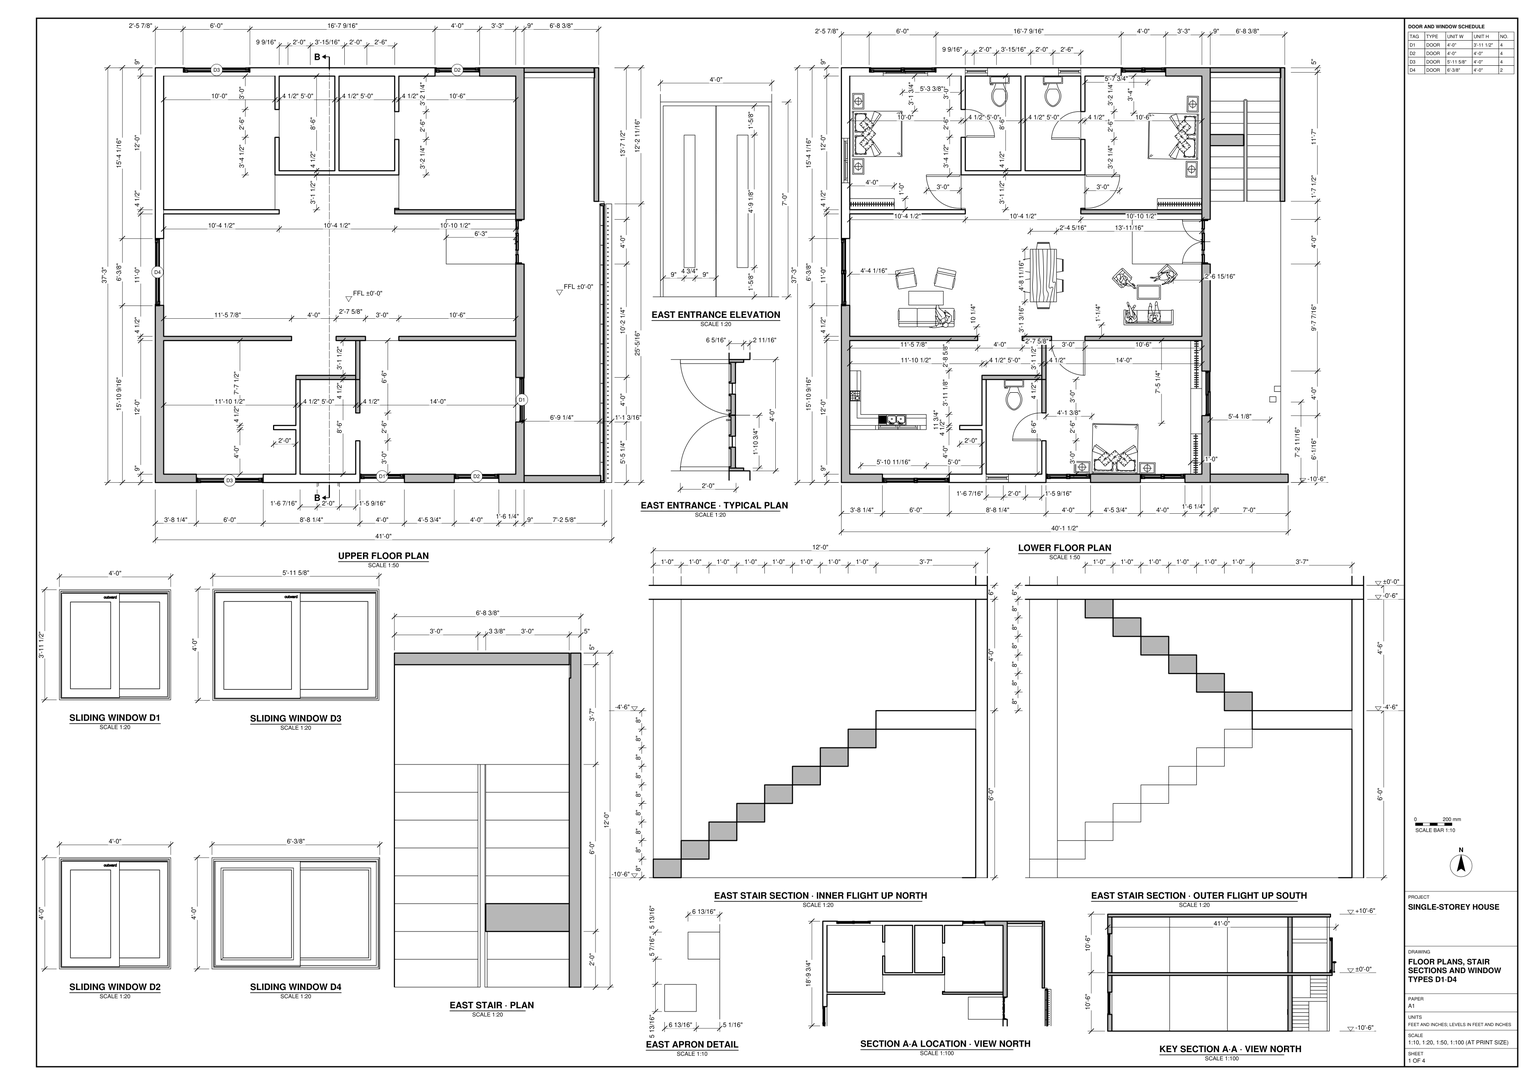
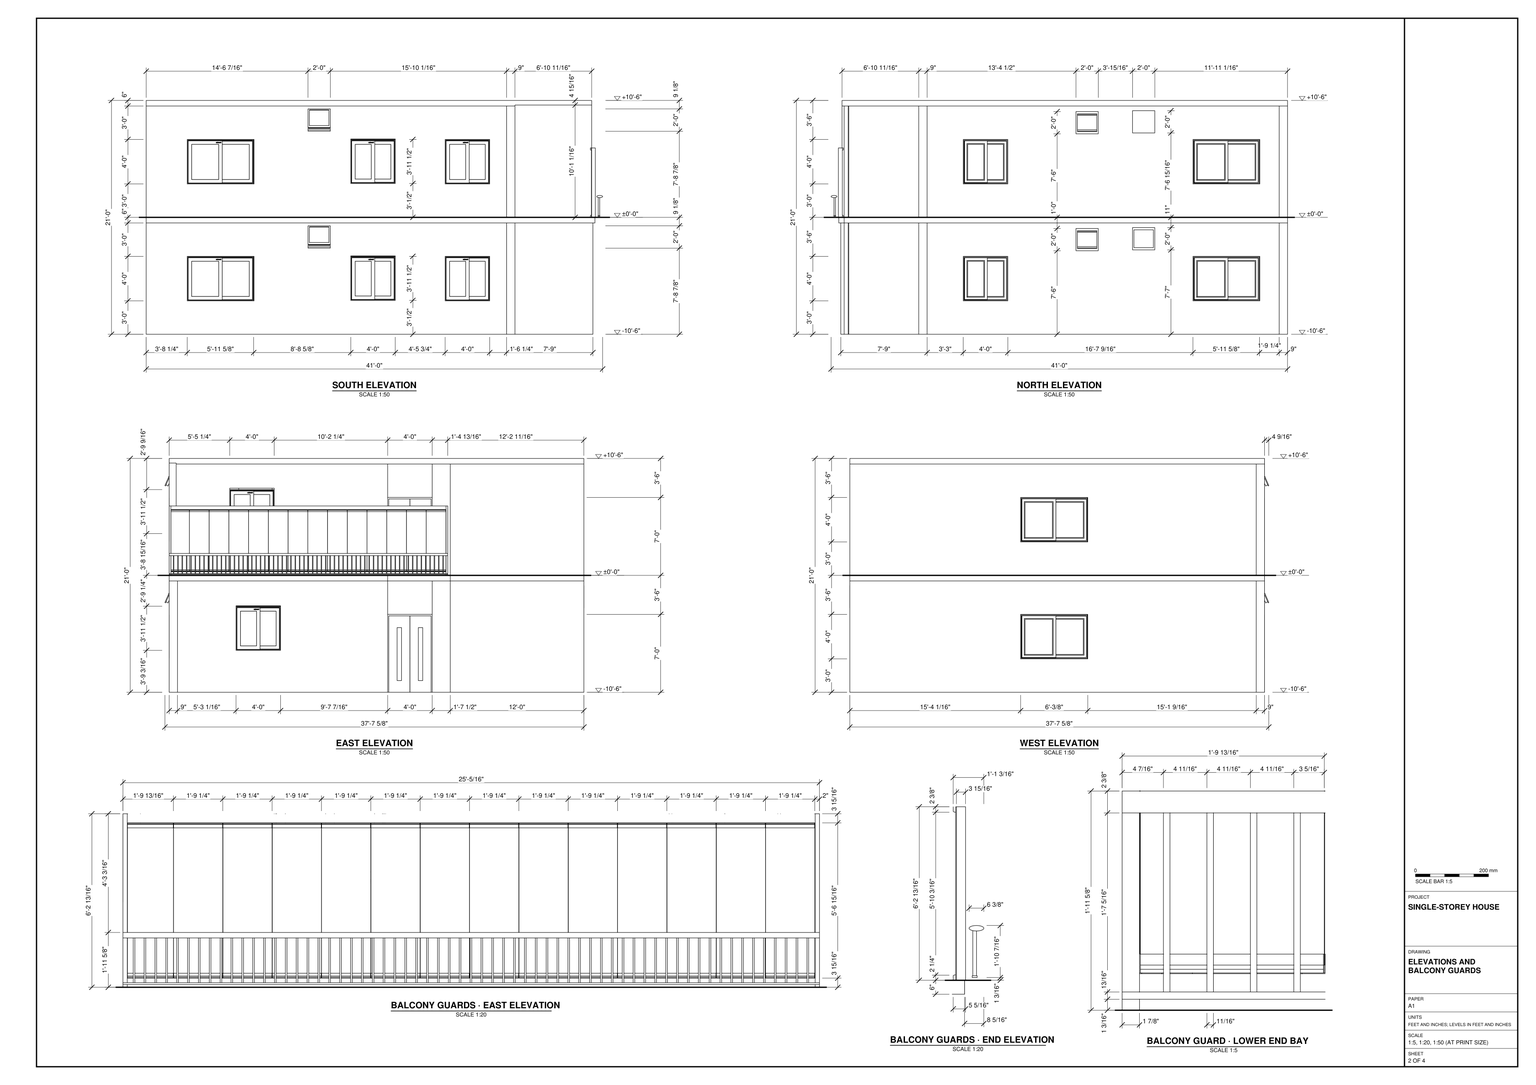
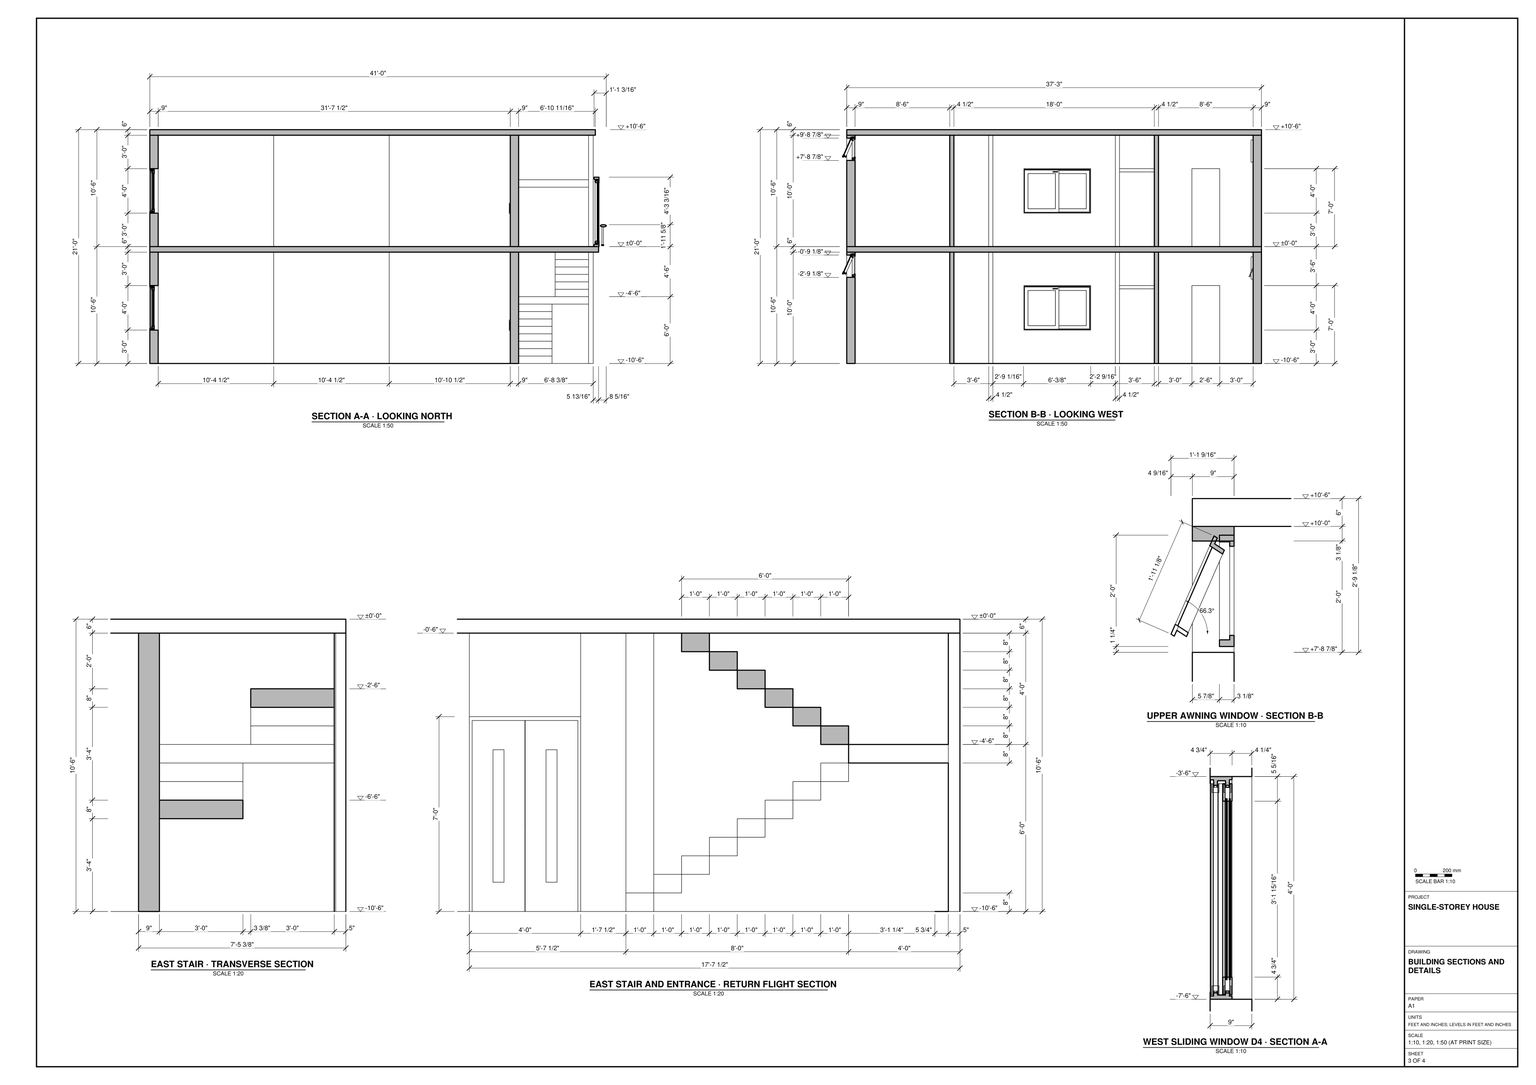
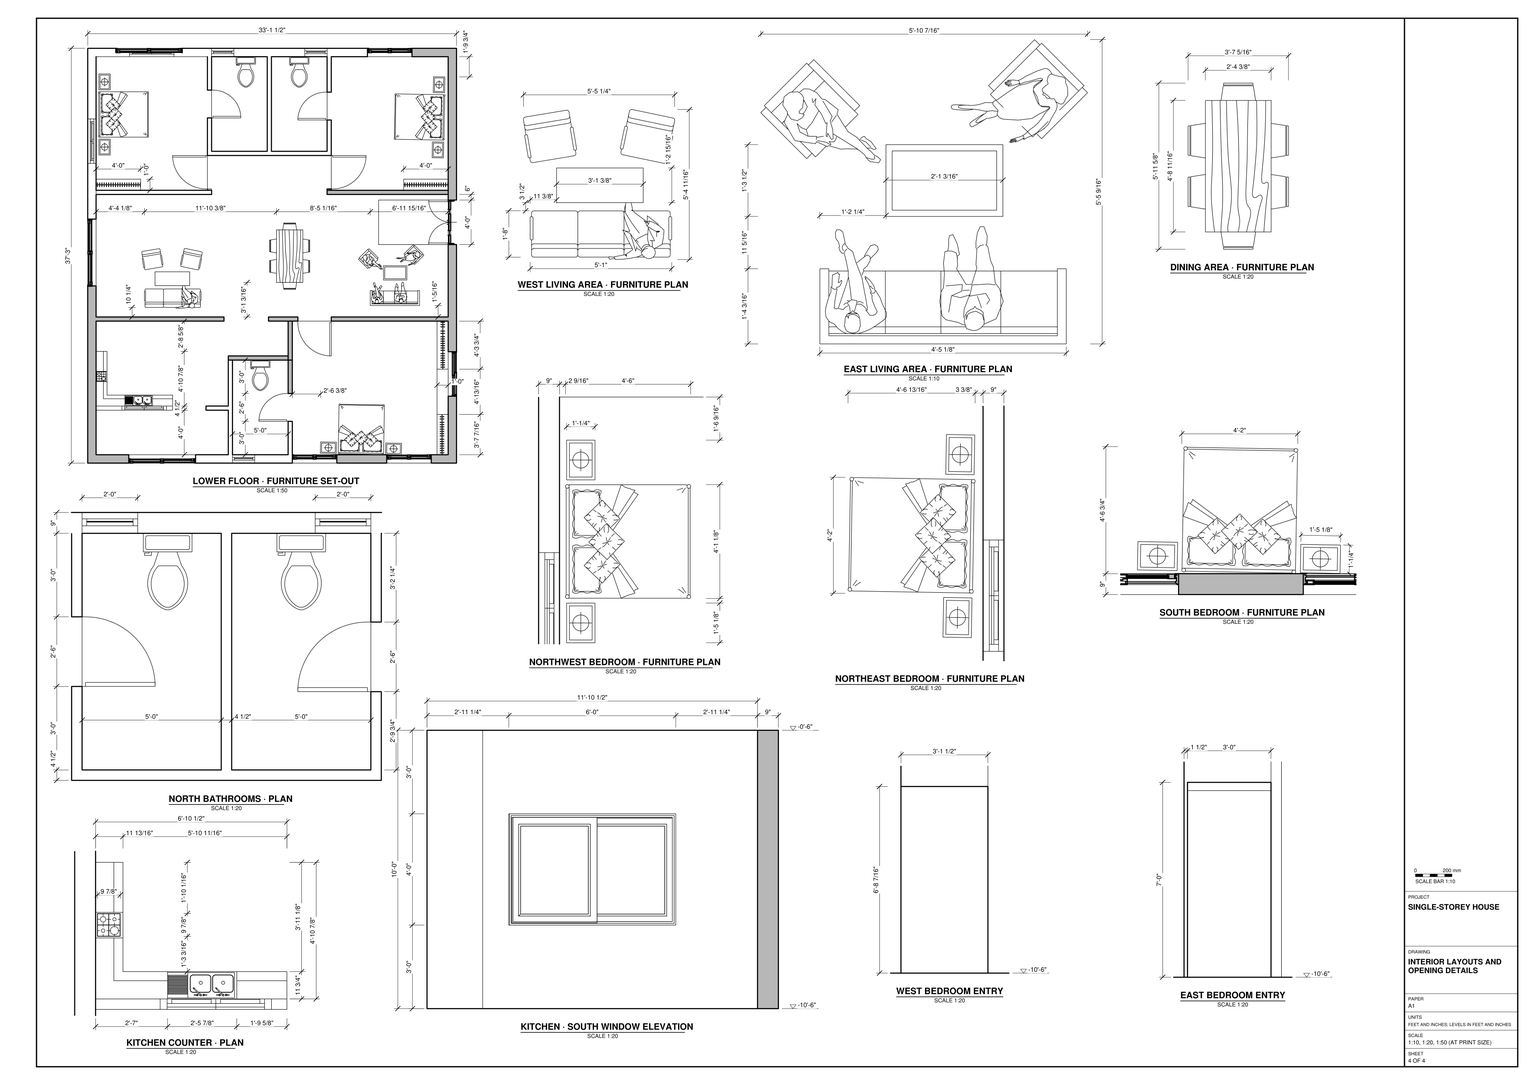
Model the house in SketchUp using task_files/diagram_01.pdf. Work in feet and inches. The overall model extents are 97'-11 5/16" along X, 37'-7 5/8" along Y and 21'-0" along Z. Use ±0'-0" as the upper floor datum. The building sections place the lower floor at -10'-6" and the top of the flat roof at +10'-6".

Set out the lower and upper walls from their respective plans, using the wall thicknesses shown. Model the floor and roof slabs, leaving access from the east stair to the balcony. Follow the stair sections for the direction of each flight and the position of the intermediate landing. Use the elevations and opening details to position the entrance doors, sliding windows and high awning windows. Include the balcony’s upper panels and lower guard.

Follow the furnished lower floor plan for the kitchen joinery, bathroom fixtures, beds, bedside furniture, dining table, chairs and living room seating. Decor and loose items may be any suitable library components. Keep shell elements such as walls, slabs and roof, and each furniture or joinery piece, in separate groups or components. Use components for repeated parts. Save one SketchUp model as output_files/house_with_its_east_return_stair_and_balcony.skp.

# SketchUp Ruby script. Lengths in inches.
U = 1.inch
M = Sketchup.active_model
def pt(a) = Geom::Point3d.new(a.map { |v| v * U })
def face(e, loops, mat)
  f = e.add_face(loops[0].map { |a| pt(a) })
  loops[1..].each { |l| e.add_face(l.map { |a| pt(a) }).erase! }
  f.material = f.back_material = mat if mat
  f
end
# faces: each face lists its corners as indices into pts; further lists are holes
def faces(e, pts, list, mat = nil) = list.each { |f| face(e, (f[0].is_a?(Array) ? f : [f]).map { |l| l.map { |i| pts[i] } }, mat) }
# xy, xz, yz: faces in a plane at the given z, y or x. An outline is a flat list of corners, or four numbers for a rectangle; further outlines are holes
def ring(l) = l.size == 4 ? [[l[0], l[1]], [l[2], l[1]], [l[2], l[3]], [l[0], l[3]]] : l.each_slice(2).to_a
def flat(e, list, mat, &to3) = list.each { |f| face(e, (f[0].is_a?(Array) ? f : [f]).map { |l| ring(l).map { |u, v| to3.(u, v) } }, mat) }
def xy(e, z, list, mat = nil) = flat(e, list, mat) { |x, y| [x, y, z] }
def xz(e, y, list, mat = nil) = flat(e, list, mat) { |x, z| [x, y, z] }
def yz(e, x, list, mat = nil) = flat(e, list, mat) { |y, z| [x, y, z] }
def lines(e, pts, list) = list.each { |a, b| e.add_line(pt(pts[a]), pt(pts[b])) }
# prism: a flat outline (further loops are holes) pulled along v
def prism(e, loops, v, mat = nil)
  f = face(e, loops, mat); d = Geom::Vector3d.new(v.map { |x| x * U })
  f.pushpull(f.normal.samedirection?(d) ? d.length : -d.length)
end
def box(e, o, s, mat = nil) = prism(e, [[o, [o[0] + s[0], o[1], o[2]], [o[0] + s[0], o[1] + s[1], o[2]], [o[0], o[1] + s[1], o[2]]]], [0, 0, s[2]], mat)
def at(x, y, z, deg = 0) = Geom::Transformation.translation(pt([x, y, z])) * Geom::Transformation.rotation(ORIGIN, Z_AXIS, deg.degrees)
def axes(o, x, y, z) = Geom::Transformation.new([*x, 0, *y, 0, *z, 0, *pt(o).to_a, 1])
def part(name) = M.definitions.add(name)
# library, detail: a bought-in or finely detailed component or shape, given as its bounding box
def library(name, o, s) = part(name).tap { |d| box(d.entities, o, s) }
def detail(e, o, s) = box(e.add_group.entities, o, s)
def put(e, d, t, mat = nil) = e.add_instance(d, t).tap { |i| i.material = mat if mat }
def group(e, t, mat = nil) = e.add_group.tap { |g| g.transformation = t; g.material = mat if mat }.entities
root = M.entities
M.materials.add("[Color M00]").color = [255, 255, 255]
M.materials.add("[Translucent Glass Gray]").color = [128, 128, 128]
M.materials["[Translucent Glass Gray]"].alpha = 0.5
c1 = part("10")
box(c1.entities,[0,0,0],[36,12,8])
c2 = library("Drawing1.dwg\#1",[0,0,0],[1199.34,447,0.01])
c3 = library("Glazed double door",[0,0,0],[62.99,7.48,78.74])
c4 = library("AS-120-mm",[0,0,0],[71.65,4.72,48])
c5 = library("AS-120-mm\#1",[0,0,0],[48,4.72,48])
c6 = library("AS-120-mm\#2",[0,0,0],[72.37,4.72,48])
c7 = library("AS-120-mm\#3",[0,0,0],[48,4.72,47.52])
c8 = part("=_UTF-8_Q_=")
xy(c8.entities,58.27,[[39.37,0,70.87,3.15]])
xy(c8.entities,59.45,[[40.55,0,69.69,2.2]])
xy(c8.entities,60.24,[[41.34,2.2,68.9,3.15]])
xy(c8.entities,75.98,[[41.34,2.2,68.9,3.15]])
xy(c8.entities,76.77,[[40.55,0,69.69,2.2]])
xy(c8.entities,77.95,[[39.37,0,70.87,3.15]])
xz(c8.entities,0,[[[39.37,58.27,70.87,77.95],[40.55,59.45,69.69,76.77]]])
xz(c8.entities,2.2,[[[40.55,59.45,69.69,76.77],[41.34,60.24,68.9,75.98]]])
xz(c8.entities,3.15,[[[39.37,58.27,70.87,77.95],[41.34,60.24,68.9,75.98]]])
yz(c8.entities,39.35,[[-9.75,60.1,-10.44,60.47,-1.17,77.83,-0.48,77.46]])
yz(c8.entities,39.37,[[0,58.27,3.15,77.95]])
yz(c8.entities,40.53,[[-7.11,60.02,-9.19,61.14,-1.03,76.42,1.05,75.31]])
yz(c8.entities,40.55,[[0,59.45,2.2,76.77]])
yz(c8.entities,41.32,[[-6.74,60.72,0.68,74.61,-1.58,75.82,-8.99,61.92]])
yz(c8.entities,41.32,[[-8.99,61.92,-1.58,75.82,-2.1,76.09,-9.51,62.2]],"[Color M00]")
yz(c8.entities,41.34,[[2.2,60.24,3.15,75.98]])
yz(c8.entities,68.875,[[-6.74,60.72,-8.99,61.92,-1.58,75.82,0.68,74.61]])
yz(c8.entities,68.875,[[-8.99,61.92,-9.51,62.2,-2.1,76.09,-1.58,75.82]],"[Color M00]")
yz(c8.entities,68.9,[[2.2,60.24,3.15,75.98]])
yz(c8.entities,69.66,[[-7.11,60.02,1.05,75.31,-1.03,76.42,-9.19,61.14]])
yz(c8.entities,69.69,[[0,59.45,2.2,76.77]])
yz(c8.entities,70.85,[[-9.75,60.1,-0.48,77.46,-1.17,77.83,-10.44,60.47]])
yz(c8.entities,70.87,[[0,58.27,3.15,77.95]])
p = [[40.53,-7.11,60.02],[69.66,-7.11,60.02],[69.66,-9.19,61.14],[40.53,-9.19,61.14],[69.66,1.05,75.31],[40.53,1.05,75.31],
  [41.32,-6.74,60.72],[68.875,-6.74,60.72],[68.875,0.68,74.61],[41.32,0.68,74.61],[70.85,-10.44,60.47],[39.35,-10.44,60.47],
  [39.35,-9.75,60.1],[70.85,-9.75,60.1],[39.35,-0.48,77.46],[70.85,-0.48,77.46],[69.66,-1.03,76.42],[40.53,-1.03,76.42],
  [39.35,-1.17,77.83],[70.85,-1.17,77.83],[68.875,-2.1,76.09],[68.875,-9.51,62.2],[41.32,-9.51,62.2],[41.32,-2.1,76.09],
  [41.32,-8.99,61.92],[68.875,-8.99,61.92],[68.875,-1.58,75.82],[41.32,-1.58,75.82]]
faces(c8.entities,p,[[0,1,2,3],[[4,1,0,5],[6,7,8,9]],[10,11,12,13],[[12,14,15,13],[2,16,17,3]],[[18,11,10,19],[20,21,22,23]],[6,24,25,7],[8,26,27,9],[4,5,17,16],
  [18,19,15,14]])
faces(c8.entities,p,[[21,25,24,22],[20,23,27,26]],"[Color M00]")
faces(c8.entities,p,[[26,27,24,25]],"[Translucent Glass Gray]")
c9 = library("FECHAMENTO VARANDA VIDRO",[23.92,27.98,0],[4.89,252.36,74.8])
c10 = part("Group111")
box(c10.entities,[868.92,435.78,90.97],[24,11.22,24])
xy(root,0,[[0,4.59,9,157.59],[9,4.59,388.5,13.59],[388.5,4.59,397.5,240.09],[1080.84,4.59,1164.84,13.59],[1144.96,91.3,1151.8,97.14],
  [0,157.59,146.85,162.09],[19.5,162.09,28.5,294.09],[388.5,288.09,397.5,451.59],[0,294.09,9,442.59],[9,294.09,133.5,298.59],
  [0,442.59,388.5,451.59]])
xy(root,120,[[[683.34,4.59,683.34,451.59,1161.22,451.59,1161.22,307.59,1167.03,307.59,1167.03,240.09,1167.01,240.09,1167.01,4.59,1164.84,4.59,1164.84,13.59,1080.84,13.59,1080.84,4.59],[1133.51,87.04,1151.18,102.47]],[1133.51,87.04,1151.18,102.47]])
xy(root,126,[[683.34,4.59,1080.84,4.59,1080.84,12.16,1163.5,12.16,1163.5,4.59,1167.01,4.59,1167.01,240.09,1167.03,240.09,1167.03,307.59,1161.22,307.59,1161.22,451.59,683.34,451.59]])
xy(root,246,[[[683.34,4.59,683.34,451.59,1163.53,451.59,1163.53,12.16,1080.84,12.16,1080.84,4.59],[1144.96,91.3,1151.8,97.14]]])
xy(root,247.04,[[1080.84,4.59,1163.5,12.16],[1163.5,4.59,1163.53,12.16]])
xy(root,252,[[683.34,4.59,1163.53,451.59]])
xz(root,4.59,[[1080.84,0,1164.84,120],[683.34,120,1167.01,120,1167.01,126,1163.5,126,1163.5,247.04,1080.84,247.04,1080.84,126,683.34,126],[683.34,246,1080.84,246,1080.84,247.04,1163.53,247.04,1163.53,252,683.34,252]])
xz(root,12.16,[[1080.84,126,1163.5,246],[1080.84,246,1163.5,247.04],[1163.5,246,1163.53,247.04]])
xz(root,13.59,[[1080.84,0,1164.84,120]])
xz(root,240.09,[[1167.01,120,1167.03,126]])
xz(root,307.59,[[1161.22,120,1167.03,126]])
xz(root,451.59,[[683.34,120,1161.22,126],[683.34,246,1163.53,252]])
yz(root,683.34,[[4.59,120,451.59,126],[4.59,246,451.59,252]])
yz(root,1080.84,[[4.59,0,13.59,120],[4.59,126,12.16,246],[4.59,246,12.16,247.04]])
yz(root,1161.22,[[307.59,120,451.59,126]])
yz(root,1163.5,[[4.59,126,12.16,247.04]])
yz(root,1163.53,[[12.16,246,451.59,246,451.59,252,4.59,252,4.59,247.04,12.16,247.04]])
yz(root,1164.84,[[4.59,0,13.59,120]])
yz(root,1167.01,[[4.59,120,240.09,126]])
yz(root,1167.03,[[240.09,120,307.59,126]])
p = [[850.42,451.63,114.97],[826.42,451.63,114.97],[826.42,451.63,90.97],[850.42,451.63,90.97],[1150,108.42,246],[1156.84,108.42,246],
  [1150,108.42,0],[1156.84,108.42,0],[1156.84,102.58,246],[1150,102.58,246],[1156.84,102.58,0],[1150,102.58,0]]
lines(root,p,[[0,1],[2,3],[1,2],[3,0],[4,5],[6,7],[8,9],[10,11],[5,8],[7,10],[9,4],[11,6]])
put(root,c1,at(1080.84,307.59,0))
put(root,c1,at(1080.84,319.59,8))
put(root,c1,at(1080.84,331.59,16))
put(root,c1,at(1080.84,343.59,24))
put(root,c1,at(1080.84,355.59,32))
put(root,c1,at(1080.84,367.59,40))
put(root,c1,at(1080.84,379.59,48))
put(root,c1,at(1080.84,391.59,56))
put(root,c1,at(1120.22,391.59,72))
put(root,c1,at(1120.22,379.59,80))
put(root,c1,at(1120.22,367.59,88))
put(root,c1,at(1120.22,355.59,96))
put(root,c1,at(1120.22,343.59,104))
put(root,c1,at(1120.22,331.59,112))
put(root,c2,at(-42.5,4.59,0))
put(root,c3,axes([1070.66,288.09,0],[0,-0.762,0],[1,0,0],[0,0,1.0668]))
put(root,c4,at(713.6,446.87,36))
put(root,c5,at(984.84,446.87,36))
put(root,c6,at(688.07,195.18,36,90))
put(root,c4,at(727.59,4.59,36))
put(root,c5,at(1005.59,8.87,36))
put(root,c7,at(903.84,8.87,36.48))
put(root,c8,axes([857.35,448.44,18.98],[0.76216,0,0],[0,1,0],[0,0,1.2192]))
put(root,c8,axes([796.41,448.48,19.93],[0.76216,0,0],[0,1,0],[0,0,1.2192]))
put(root,c8,axes([827.78,10.44,23.07],[0.76216,0,0],[0,1,0],[0,0,1.2192]))
put(root,c5,at(984.84,446.87,162))
put(root,c8,axes([857.35,448.44,144.98],[0.76216,0,0],[0,1,0],[0,0,1.2192]))
put(root,c3,axes([1070.66,288.09,126],[0,-0.762,0],[1,0,0],[0,0,1.0668]))
put(root,c5,at(1005.59,8.87,162))
put(root,c6,at(688.07,195.18,162,90))
put(root,c4,at(727.59,4.59,162))
put(root,c4,at(713.6,446.87,162))
put(root,c8,axes([827.78,10.44,149.07],[0.76216,0,0],[0,1,0],[0,0,1.2192]))
put(root,c7,at(903.84,8.87,162.48))
put(root,c9,axes([1097.46,-28.71,126],[2.7027,0,0],[0,1.19,0],[0,0,1]))
put(root,c7,at(1080.84,76.68,45.21,90))
put(root,c7,at(1080.84,69.85,170.95,90))
put(root,c10,at(-42.5,4.59,0))
g1 = group(root,at(683.34,4.59,0))
xy(g1,0,[[0,0,0,447,388.5,447,388.5,438,262.5,438,262.5,399.75,258,399.75,258,438,198,438,198,336,258,336,258,369.75,262.5,369.75,262.5,331.5,129,331.5,129,372,133.5,372,133.5,336,193.5,336,193.5,438,133.5,438,133.5,402,129,402,129,438,9,438,9,157.5,146.853,157.5,146.853,153,9,153,9,9,151.5,9,151.5,57,127.5,57,127.5,61.5,151.5,61.5,151.5,111,156,111,156,9,216,9,216,45,220.5,45,220.5,9,388.5,9,388.5,235.5,397.5,235.5,397.5,0],[9,9,9,153,146.853,153,146.853,157.5,9,157.5,9,289.5,133.5,289.5,133.5,294,129,294,129,331.5,262.5,331.5,262.5,295.5,258,295.5,258,289.5,388.5,289.5,388.5,283.5,313.5,283.5,313.5,235.5,388.5,235.5,388.5,157.5,262.5,157.5,262.5,153,226.5,153,226.5,157.5,194.853,157.5,194.853,153,216,153,216,115.5,151.5,115.5,151.5,61.5,127.5,61.5,127.5,57,151.5,57,151.5,9],[216,75,220.5,111],[151.5,111,156,111.011],[156,111,216,111.011],
  [216,111,220.5,111.011],[151.5,111.011,216,115.5],[216,111.011,220.5,153],[194.853,153,226.5,157.5],[262.5,153,388.5,157.5],
  [313.5,235.5,388.5,283.5],[388.5,283.5,397.5,447],[9,289.5,133.5,294],[258,289.5,388.5,294],[258,294,262.5,295.5],
  [133.5,336,193.5,438],[198,336,258,438],[397.5,436.228,472.875,442],[472.875,436.228,473.5,442],[472.875,442,473.5,447]])
xy(g1,36,[[44.25,0,116.25,9],[322.251,0,370.251,9],[0,190.957,9,262.957],[301.5,438,349.5,447]])
xy(g1,36.468,[[220.5,0,268.5,9]])
xy(g1,45.21,[[388.5,72.087,397.5,120.087]])
xy(g1,64,[[397.5,399,472.875,442]])
xy(g1,72,[[397.5,399,472.875,442]])
xy(g1,80.449,[[129,294,133.5,331.5]])
xy(g1,84,[[44.25,0,116.25,9],[322.251,0,370.251,9],[216,45,220.5,75],[226.5,153,262.5,157.5],[0,190.957,9,262.957],
  [388.5,235.5,397.5,283.5],[258,295.5,262.5,331.5],[258,369.75,262.5,399.75],[129,372,133.5,402],[301.5,438,349.5,447]])
xy(g1,84.468,[[220.5,0,268.5,9]])
xy(g1,90.023,[[204.02,438,228.02,447]])
xy(g1,92.85,[[174.453,0,198.453,9]])
xy(g1,93.21,[[388.5,72.087,397.5,120.087]])
xy(g1,114.023,[[204.02,438,228.02,447]])
xy(g1,116.85,[[174.453,0,198.453,9]])
xy(g1,120,[[0,0,388.5,9],[388.5,0,397.5,235.5],[0,9,9,447],[151.5,9,156,111],[216,9,220.5,75],
  [127.5,57,151.5,61.5],[216,75,220.5,111],[151.5,111.011,216,115.5],[216,111.011,220.5,153],[9,153,146.853,157.5],
  [194.853,153,388.5,157.5],[388.5,235.5,397.5,283.5],[388.5,283.5,397.5,447],[9,289.5,133.5,294],[258,289.5,388.5,294],
  [129,294,133.5,331.5],[258,294,262.5,331.5],[472.875,303,472.875,436.228,473.5,436.228,473.5,447,477.875,447,477.875,303],[129,331.5,133.5,438],[133.5,331.5,258,336],
  [258,331.5,262.5,438],[193.5,336,198,438],[9,438,388.5,447],[397.5,442,472.875,447]])
xz(g1,0,[[[0,0,388.5,120],[44.25,36,116.25,84],[322.251,36,370.251,84],[220.5,36.468,268.5,84.468],[174.453,92.85,198.453,116.85]],[388.5,0,397.5,120]])
xz(g1,9,[[[9,0,151.5,120],[44.25,36,116.25,84]],[[156,0,216,120],[174.453,92.85,198.453,116.85]],[[220.5,0,220.5,36.468,268.5,36.468,268.5,84.468,220.5,84.468,220.5,120,388.5,120,388.5,0],[322.251,36,370.251,84]]])
xz(g1,45,[[216,0,220.5,84]])
xz(g1,57,[[127.5,0,151.5,120]])
xz(g1,61.5,[[127.5,0,151.5,120]])
xz(g1,72.087,[[388.5,45.21,397.5,93.21]])
xz(g1,75,[[216,0,220.5,84]])
xz(g1,111,[[151.5,0,156,120],[216,0,220.5,120]])
xz(g1,111.011,[[151.5,0,156,120],[156,0,216,120],[216,0,220.5,120]])
xz(g1,115.5,[[151.5,0,216,120]])
xz(g1,120.087,[[388.5,45.21,397.5,93.21]])
xz(g1,153,[[9,0,146.853,120],[194.853,0,216,120],[216,0,220.5,120],[220.5,0,226.5,0,226.5,84,262.5,84,262.5,0,388.5,0,388.5,120,220.5,120]])
xz(g1,157.5,[[9,0,146.853,120],[194.853,0,194.853,120,388.5,120,388.5,0,262.5,0,262.5,84,226.5,84,226.5,0]])
xz(g1,190.957,[[0,36,9,84]])
xz(g1,235.5,[[388.5,0,397.5,84],[388.5,84,397.5,120]])
xz(g1,262.957,[[0,36,9,84]])
xz(g1,283.5,[[388.5,0,397.5,84],[388.5,84,397.5,120]])
xz(g1,289.5,[[9,0,133.5,120],[258,0,388.5,120]])
xz(g1,294,[[9,0,129,120],[129,0,133.5,80.449],[258,0,262.5,120],[262.5,0,388.5,120],[129,80.449,133.5,120]])
xz(g1,295.5,[[258,0,262.5,84]])
xz(g1,303,[[472.875,0,477.875,120]])
xz(g1,331.5,[[129,0,262.5,0,262.5,84,258,84,258,120,133.5,120,133.5,80.449,129,80.449]])
xz(g1,336,[[133.5,0,193.5,120],[198,0,258,120]])
xz(g1,369.75,[[258,0,262.5,84]])
xz(g1,372,[[129,0,133.5,84]])
xz(g1,399,[[397.5,64,472.875,72]])
xz(g1,399.75,[[258,0,262.5,84]])
xz(g1,402,[[129,0,133.5,84]])
xz(g1,436.228,[[472.875,0,473.5,120]])
xz(g1,438,[[133.5,0,193.5,120],[[198,0,258,120],[204.02,90.023,228.02,114.023]],[[262.5,0,388.5,120],[301.5,36,349.5,84]]])
xz(g1,442,[[397.5,0,472.875,64],[397.5,72,472.875,120]])
xz(g1,447,[[0,0,9,120],[[9,0,388.5,120],[29.907,36,101.907,84],[301.5,36,349.5,84],[204.02,90.023,228.02,114.023]],[388.5,0,397.5,120],[397.5,0,472.875,120],[473.5,0,477.875,120]])
yz(g1,0,[[0,0,9,120],[[9,0,447,120],[190.957,36,262.957,84]]])
yz(g1,9,[[9,0,153,120],[[157.5,0,289.5,120],[190.957,36,262.957,84]],[294,0,438,120]])
yz(g1,44.25,[[0,36,9,84]])
yz(g1,116.25,[[0,36,9,84]])
yz(g1,127.5,[[57,0,61.5,120]])
yz(g1,129,[[331.5,0,331.5,120,438,120,438,0,402,0,402,84,372,84,372,0],[294,80.449,331.5,120]])
yz(g1,133.5,[[289.5,0,294,120],[336,0,372,0,372,84,402,84,402,0,438,0,438,120,336,120],[294,80.449,331.5,84],[294,84,331.5,120]])
yz(g1,146.853,[[153,0,157.5,120]])
yz(g1,151.5,[[9,0,57,120],[61.5,0,111,120],[111.011,0,115.5,120]])
yz(g1,156,[[9,0,111,120]])
yz(g1,174.453,[[0,92.85,9,116.85]])
yz(g1,193.5,[[336,0,438,120]])
yz(g1,194.853,[[153,0,157.5,120]])
yz(g1,198,[[336,0,438,120]])
yz(g1,198.453,[[0,92.85,9,116.85]])
yz(g1,204.02,[[438,90.023,447,114.023]])
yz(g1,216,[[9,0,9,120,75,120,75,84,45,84,45,0],[75,0,111,120],[111.011,0,115.5,120],[115.5,0,153,120]])
yz(g1,220.5,[[9,0,45,0,45,84,75,84,75,120,9,120],[75,0,111,120],[111.011,0,115.5,120],[115.5,0,153,120],[0,36.468,9,84.468]])
yz(g1,226.5,[[153,0,157.5,84]])
yz(g1,228.02,[[438,90.023,447,114.023]])
yz(g1,258,[[289.5,0,294,120],[294,0,294,120,331.5,120,331.5,84,295.5,84,295.5,0],[336,0,336,120,438,120,438,0,399.75,0,399.75,84,369.75,84,369.75,0]])
yz(g1,262.5,[[153,0,157.5,84],[294,0,295.5,0,295.5,84,331.5,84,331.5,120,294,120],[331.5,0,369.75,0,369.75,84,399.75,84,399.75,0,438,0,438,120,331.5,120]])
yz(g1,268.5,[[0,36.468,9,84.468]])
yz(g1,301.5,[[438,36,447,84]])
yz(g1,322.251,[[0,36,9,84]])
yz(g1,349.5,[[438,36,447,84]])
yz(g1,370.251,[[0,36,9,84]])
yz(g1,388.5,[[[9,0,153,120],[72.087,45.21,120.087,93.21]],[157.5,0,235.5,120],[283.5,0,289.5,120],[289.5,0,294,120],[294,0,438,120],
  [235.5,84,283.5,120]])
yz(g1,397.5,[[[0,0,235.5,120],[72.087,45.21,120.087,93.21]],[283.5,0,303,120],[303,0,315,120],[315,0,442,0,442,64,399,64,399,72,442,72,442,120,315,120],[442,0,447,120],
  [399,64,442,72],[235.5,84,283.5,120]])
yz(g1,472.875,[[303,0,436.228,0,436.228,64,399,64,399,72,436.228,72,436.228,120,303,120],[442,0,447,120],[399,64,436.228,72],[436.228,64,442,72]])
yz(g1,473.5,[[436.228,0,442,120],[442,0,447,120]])
yz(g1,477.875,[[303,0,447,120]])
put(root,c10,at(-42.5,4.59,126))
g2 = group(root,at(683.34,4.59,126))
xy(g2,0,[[0,0,0,447,388.5,447,388.5,438,262.5,438,262.5,399.75,258,399.75,258,438,198,438,198,336,258,336,258,369.75,262.5,369.75,262.5,331.5,129,331.5,129,372,133.5,372,133.5,336,193.5,336,193.5,438,133.5,438,133.5,402,129,402,129,438,9,438,9,157.5,146.853,157.5,146.853,153,9,153,9,9,151.5,9,151.5,57,127.5,57,127.5,61.5,151.5,61.5,151.5,111,156,111,156,9,216,9,216,45,220.5,45,220.5,9,388.5,9,388.5,235.5,397.5,235.5,397.5,0],[9,9,9,153,146.853,153,146.853,157.5,9,157.5,9,289.5,133.5,289.5,133.5,294,129,294,129,331.5,262.5,331.5,262.5,295.5,258,295.5,258,289.5,388.5,289.5,388.5,283.5,313.5,283.5,313.5,235.5,388.5,235.5,388.5,157.5,262.5,157.5,262.5,153,226.5,153,226.5,157.5,194.853,157.5,194.853,153,216,153,216,115.5,151.5,115.5,151.5,61.5,127.5,61.5,127.5,57,151.5,57,151.5,9],[216,75,220.5,111],[151.5,111,156,111.011],[156,111,216,111.011],
  [216,111,220.5,111.011],[151.5,111.011,216,115.5],[216,111.011,220.5,153],[194.853,153,226.5,157.5],[262.5,153,388.5,157.5],
  [313.5,235.5,388.5,283.5],[388.5,283.5,397.5,447],[9,289.5,133.5,294],[258,289.5,388.5,294],[258,294,262.5,295.5],
  [133.5,336,193.5,438],[198,336,258,438],[397.5,436.228,472.875,442],[472.875,436.228,473.5,442],[472.875,442,473.5,447]])
xy(g2,36,[[44.25,0,116.25,9],[322.251,0,370.251,9],[0,190.957,9,262.957],[301.5,438,349.5,447]])
xy(g2,36.468,[[220.5,0,268.5,9]])
xy(g2,44.948,[[388.5,65.259,397.5,113.259]])
xy(g2,64,[[397.5,399,472.875,442]])
xy(g2,72,[[397.5,399,472.875,442]])
xy(g2,80.449,[[129,294,133.5,331.5]])
xy(g2,84,[[44.25,0,116.25,9],[322.251,0,370.251,9],[216,45,220.5,75],[226.5,153,262.5,157.5],[0,190.957,9,262.957],
  [388.5,235.5,397.5,283.5],[258,295.5,262.5,331.5],[258,369.75,262.5,399.75],[129,372,133.5,402],[301.5,438,349.5,447]])
xy(g2,84.468,[[220.5,0,268.5,9]])
xy(g2,90.023,[[204.02,438,228.02,447]])
xy(g2,92.85,[[174.453,0,198.453,9]])
xy(g2,93.951,[[388.5,65.259,397.5,113.259]])
xy(g2,114.023,[[204.02,438,228.02,447]])
xy(g2,116.85,[[174.453,0,198.453,9]])
xy(g2,120,[[0,0,388.5,9],[388.5,0,397.5,235.5],[0,9,9,447],[151.5,9,156,111],[216,9,220.5,75],
  [127.5,57,151.5,61.5],[216,75,220.5,111],[151.5,111.011,216,115.5],[216,111.011,220.5,153],[9,153,146.853,157.5],
  [194.853,153,388.5,157.5],[388.5,235.5,397.5,283.5],[388.5,283.5,397.5,447],[9,289.5,133.5,294],[258,289.5,388.5,294],
  [129,294,133.5,331.5],[258,294,262.5,331.5],[472.875,303,472.875,436.228,473.5,436.228,473.5,447,477.875,447,477.875,303],[129,331.5,133.5,438],[133.5,331.5,258,336],
  [258,331.5,262.5,438],[193.5,336,198,438],[9,438,388.5,447],[397.5,442,472.875,447]])
xz(g2,0,[[[0,0,388.5,120],[44.25,36,116.25,84],[322.251,36,370.251,84],[220.5,36.468,268.5,84.468],[174.453,92.85,198.453,116.85]],[388.5,0,397.5,120]])
xz(g2,9,[[[9,0,151.5,120],[44.25,36,116.25,84]],[[156,0,216,120],[174.453,92.85,198.453,116.85]],[[220.5,0,220.5,36.468,268.5,36.468,268.5,84.468,220.5,84.468,220.5,120,388.5,120,388.5,0],[322.251,36,370.251,84]]])
xz(g2,45,[[216,0,220.5,84]])
xz(g2,57,[[127.5,0,151.5,120]])
xz(g2,61.5,[[127.5,0,151.5,120]])
xz(g2,65.259,[[388.5,44.948,397.5,45.951],[388.5,45.951,397.5,92.948],[388.5,92.948,397.5,93.951]])
xz(g2,75,[[216,0,220.5,84]])
xz(g2,111,[[151.5,0,156,120],[216,0,220.5,120]])
xz(g2,111.011,[[151.5,0,156,120],[156,0,216,120],[216,0,220.5,120]])
xz(g2,113.259,[[388.5,44.948,397.5,45.951],[388.5,45.951,397.5,92.948],[388.5,92.948,397.5,93.951]])
xz(g2,115.5,[[151.5,0,216,120]])
xz(g2,153,[[9,0,146.853,120],[194.853,0,216,120],[216,0,220.5,120],[220.5,0,226.5,0,226.5,84,262.5,84,262.5,0,388.5,0,388.5,120,220.5,120]])
xz(g2,157.5,[[9,0,146.853,120],[194.853,0,194.853,120,388.5,120,388.5,0,262.5,0,262.5,84,226.5,84,226.5,0]])
xz(g2,190.957,[[0,36,9,84]])
xz(g2,235.5,[[388.5,0,397.5,84],[388.5,84,397.5,120]])
xz(g2,262.957,[[0,36,9,84]])
xz(g2,283.5,[[388.5,0,397.5,84],[388.5,84,397.5,120]])
xz(g2,289.5,[[9,0,133.5,120],[258,0,388.5,120]])
xz(g2,294,[[9,0,129,120],[129,0,133.5,80.449],[258,0,262.5,120],[262.5,0,388.5,120],[129,80.449,133.5,120]])
xz(g2,295.5,[[258,0,262.5,84]])
xz(g2,303,[[472.875,0,477.875,120]])
xz(g2,331.5,[[129,0,262.5,0,262.5,84,258,84,258,120,133.5,120,133.5,80.449,129,80.449]])
xz(g2,336,[[133.5,0,193.5,120],[198,0,258,120]])
xz(g2,369.75,[[258,0,262.5,84]])
xz(g2,372,[[129,0,133.5,84]])
xz(g2,399,[[397.5,64,472.875,72]])
xz(g2,399.75,[[258,0,262.5,84]])
xz(g2,402,[[129,0,133.5,84]])
xz(g2,436.228,[[472.875,0,473.5,120]])
xz(g2,438,[[133.5,0,193.5,120],[[198,0,258,120],[204.02,90.023,228.02,114.023]],[[262.5,0,388.5,120],[301.5,36,349.5,84]]])
xz(g2,442,[[397.5,0,472.875,64],[397.5,72,472.875,120]])
xz(g2,447,[[0,0,9,120],[[9,0,388.5,120],[29.907,36,101.907,84],[301.5,36,349.5,84],[204.02,90.023,228.02,114.023]],[388.5,0,397.5,120],[397.5,0,472.875,120],[473.5,0,477.875,120]])
yz(g2,0,[[0,0,9,120],[[9,0,447,120],[190.957,36,262.957,84]]])
yz(g2,9,[[9,0,153,120],[[157.5,0,289.5,120],[190.957,36,262.957,84]],[294,0,438,120]])
yz(g2,44.25,[[0,36,9,84]])
yz(g2,116.25,[[0,36,9,84]])
yz(g2,127.5,[[57,0,61.5,120]])
yz(g2,129,[[331.5,0,331.5,120,438,120,438,0,402,0,402,84,372,84,372,0],[294,80.449,331.5,120]])
yz(g2,133.5,[[289.5,0,294,120],[336,0,372,0,372,84,402,84,402,0,438,0,438,120,336,120],[294,80.449,331.5,84],[294,84,331.5,120]])
yz(g2,146.853,[[153,0,157.5,120]])
yz(g2,151.5,[[9,0,57,120],[61.5,0,111,120],[111.011,0,115.5,120]])
yz(g2,156,[[9,0,111,120]])
yz(g2,174.453,[[0,92.85,9,116.85]])
yz(g2,193.5,[[336,0,438,120]])
yz(g2,194.853,[[153,0,157.5,120]])
yz(g2,198,[[336,0,438,120]])
yz(g2,198.453,[[0,92.85,9,116.85]])
yz(g2,204.02,[[438,90.023,447,114.023]])
yz(g2,216,[[9,0,9,120,75,120,75,84,45,84,45,0],[75,0,111,120],[111.011,0,115.5,120],[115.5,0,153,120]])
yz(g2,220.5,[[9,0,45,0,45,84,75,84,75,120,9,120],[75,0,111,120],[111.011,0,115.5,120],[115.5,0,153,120],[0,36.468,9,84.468]])
yz(g2,226.5,[[153,0,157.5,84]])
yz(g2,228.02,[[438,90.023,447,114.023]])
yz(g2,258,[[289.5,0,294,120],[294,0,294,120,331.5,120,331.5,84,295.5,84,295.5,0],[336,0,336,120,438,120,438,0,399.75,0,399.75,84,369.75,84,369.75,0]])
yz(g2,262.5,[[153,0,157.5,84],[294,0,295.5,0,295.5,84,331.5,84,331.5,120,294,120],[331.5,0,369.75,0,369.75,84,399.75,84,399.75,0,438,0,438,120,331.5,120]])
yz(g2,268.5,[[0,36.468,9,84.468]])
yz(g2,301.5,[[438,36,447,84]])
yz(g2,322.251,[[0,36,9,84]])
yz(g2,349.5,[[438,36,447,84]])
yz(g2,370.251,[[0,36,9,84]])
yz(g2,388.5,[[[9,0,153,120],[65.259,44.948,113.259,93.951]],[157.5,0,235.5,120],[283.5,0,289.5,120],[289.5,0,294,120],[294,0,438,120],
  [235.5,84,283.5,120]])
yz(g2,397.5,[[[0,0,235.5,120],[65.259,44.948,113.259,93.951]],[283.5,0,303,120],[303,0,315,120],[315,0,442,0,442,64,399,64,399,72,442,72,442,120,315,120],[442,0,447,120],
  [399,64,442,72],[235.5,84,283.5,120]])
yz(g2,472.875,[[303,0,436.228,0,436.228,64,399,64,399,72,436.228,72,436.228,120,303,120],[442,0,447,120],[399,64,436.228,72],[436.228,64,442,72]])
yz(g2,473.5,[[436.228,0,442,120],[442,0,447,120]])
yz(g2,477.875,[[303,0,447,120]])
